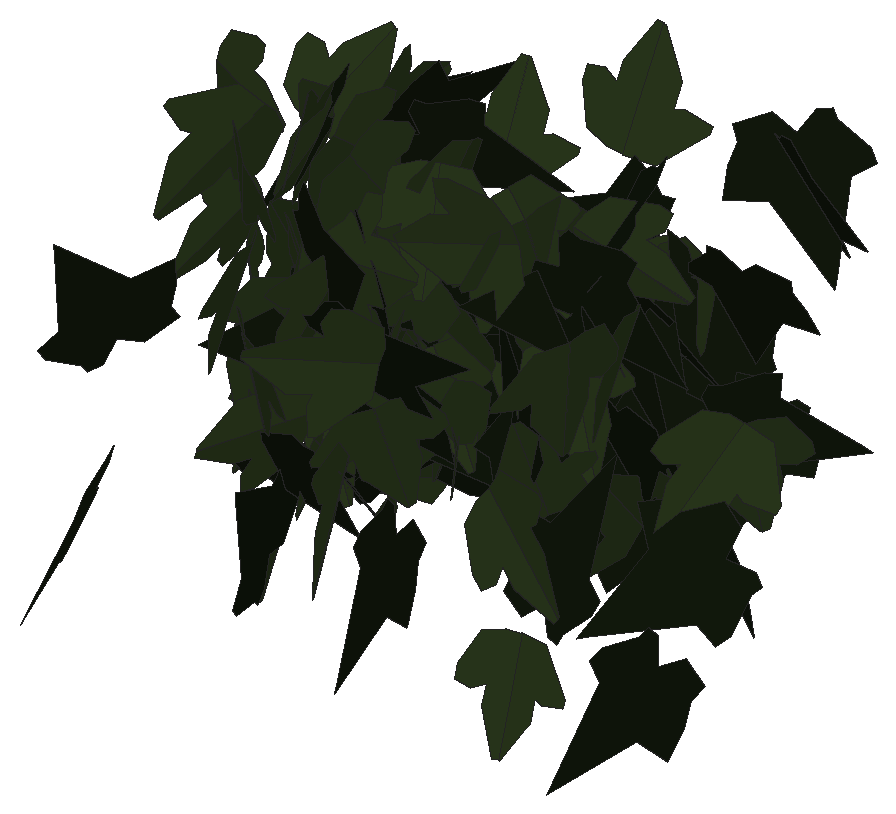
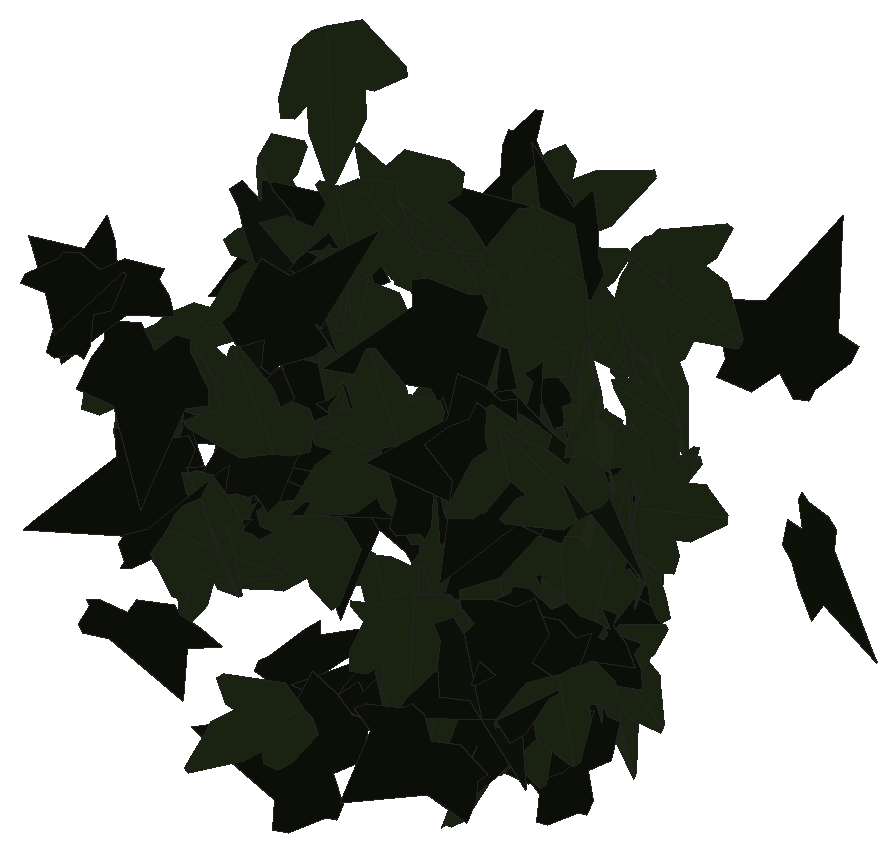
# SketchUp Ruby script. Lengths in inches.
U = 1.inch
M = Sketchup.active_model
def pt(a) = Geom::Point3d.new(a.map { |v| v * U })
def face(e, loops, mat)
  f = e.add_face(loops[0].map { |a| pt(a) })
  loops[1..].each { |l| e.add_face(l.map { |a| pt(a) }).erase! }
  f.material = f.back_material = mat if mat
  f
end
# faces: each face lists its corners as indices into pts; further lists are holes
def faces(e, pts, list, mat = nil) = list.each { |f| face(e, (f[0].is_a?(Array) ? f : [f]).map { |l| l.map { |i| pts[i] } }, mat) }
# xy, xz, yz: faces in a plane at the given z, y or x. An outline is a flat list of corners, or four numbers for a rectangle; further outlines are holes
def ring(l) = l.size == 4 ? [[l[0], l[1]], [l[2], l[1]], [l[2], l[3]], [l[0], l[3]]] : l.each_slice(2).to_a
def flat(e, list, mat, &to3) = list.each { |f| face(e, (f[0].is_a?(Array) ? f : [f]).map { |l| ring(l).map { |u, v| to3.(u, v) } }, mat) }
def xy(e, z, list, mat = nil) = flat(e, list, mat) { |x, y| [x, y, z] }
def xz(e, y, list, mat = nil) = flat(e, list, mat) { |x, z| [x, y, z] }
def yz(e, x, list, mat = nil) = flat(e, list, mat) { |y, z| [x, y, z] }
def lines(e, pts, list) = list.each { |a, b| e.add_line(pt(pts[a]), pt(pts[b])) }
# prism: a flat outline (further loops are holes) pulled along v
def prism(e, loops, v, mat = nil)
  f = face(e, loops, mat); d = Geom::Vector3d.new(v.map { |x| x * U })
  f.pushpull(f.normal.samedirection?(d) ? d.length : -d.length)
end
def box(e, o, s, mat = nil) = prism(e, [[o, [o[0] + s[0], o[1], o[2]], [o[0] + s[0], o[1] + s[1], o[2]], [o[0], o[1] + s[1], o[2]]]], [0, 0, s[2]], mat)
def at(x, y, z, deg = 0) = Geom::Transformation.translation(pt([x, y, z])) * Geom::Transformation.rotation(ORIGIN, Z_AXIS, deg.degrees)
def axes(o, x, y, z) = Geom::Transformation.new([*x, 0, *y, 0, *z, 0, *pt(o).to_a, 1])
def part(name) = M.definitions.add(name)
# library, detail: a bought-in or finely detailed component or shape, given as its bounding box
def library(name, o, s) = part(name).tap { |d| box(d.entities, o, s) }
def detail(e, o, s) = box(e.add_group.entities, o, s)
def put(e, d, t, mat = nil) = e.add_instance(d, t).tap { |i| i.material = mat if mat }
def group(e, t, mat = nil) = e.add_group.tap { |g| g.transformation = t; g.material = mat if mat }.entities
root = M.entities
M.materials.add("efeu1").color = [18, 25, 13]
M.materials.add("efeu2").color = [43, 57, 29]
c1 = part("ivyleaf_10")
p = [[0,0.5,-0.03],[-0.0625,2.02,-0.43],[-0.19,2.01,-0.46],[-0.54,1.05,-0.29],[-0.52,0.625,-0.18],[-0.83,0.76,-0.28],
  [-1.16,0.64,-0.33],[-1.15,0.33,-0.24],[-0.77,-0.39,0.02],[-0.3,-0.51,0.16],[0.04,-0.48,0.23],[-0.02,2.01,-0.4375],
  [-0.06,2.01,-0.43],[0.04,-0.49,0.23],[0.67,-0.49,0.14],[1.38,0.36,-0.2],[1.375,0.51,-0.24],[0.81,0.65,-0.19],
  [0.62,0.59,-0.15],[0.6,1.09,-0.28],[0.5,1.23,-0.31]]
faces(c1.entities,p,[[0,1,2,3,4,5,6,7,8,9,10],[11,12,0,13,14,15,16,17,18,19,20]],"efeu2")
c2 = part("ivyleaf_9")
p = [[1.54,2.16,1.25],[1.36,2.04,1.19],[-0.21,0.99,0.68],[-0.71,1.11,0.82],[-0.85,0.86,0.67],[-0.8,0.17,0.21],
  [-0.9,-0.01,0.1],[-0.67,-0.16,-0.02],[-0.08,-0.08,-0.05],[-0.03,-0.6,-0.4],[0.65,-0.88,-0.66],[0.83,-0.6,-0.49],
  [1.29,-0.42,-0.43],[1.8125,-0.07,-0.26],[1.21,0.44,0.15]]
faces(c2.entities,p,[[0,1,2,3,4,5,6,7,8,9,10,11,12,13,14]],"efeu1")
put(root,c1,axes([532.08,134.94,161.78],[-0.002,-0.30282,0.71041],[0.08269,-0.70641,-0.30089],[0.76782,0.07529,0.03425]))
put(root,c1,axes([531.67,135.35,163.72],[-0.12036,0.03541,-0.73913],[0.60153,-0.43146,-0.11862],[-0.43098,-0.61209,0.04086]))
put(root,c1,axes([532.1875,137.11,159.68],[0.41197,0.62153,-0.13019],[-0.08175,-0.10199,-0.74558],[-0.62974,0.41984,0.01161]))
put(root,c1,axes([532.44,135.95,160.75],[-0.0692,-0.6273,-0.50852],[-0.05873,-0.50512,0.6311],[-0.80539,0.09073,-0.00233]))
put(root,c2,axes([532.82,136.0625,163.02],[-0.57789,0.4659,-0.23379],[0.18175,-0.14706,-0.74231],[-0.48856,-0.6058,0.00039]))
put(root,c1,axes([532.21,136.84,162.81],[0.52698,0.21784,-0.49866],[0.45176,0.21184,0.56996],[0.30336,-0.69389,0.01746]))
put(root,c2,axes([532.9,130.41,159.11],[-0.55637,0.44266,-0.4062],[0.31798,-0.25276,-0.71098],[-0.50974,-0.64082,-0.00016]))
put(root,c1,axes([532.81,135.01,158.96],[0.02058,-0.62016,0.37202],[0.0037,-0.37207,-0.62046],[0.72318,0.01955,-0.00741]))
put(root,c1,axes([532.47,134.8125,161.05],[-0.14719,0.19766,-0.6896],[0.32766,-0.60772,-0.24413],[-0.63816,-0.35762,0.0337]))
put(root,c1,axes([533.27,135.22,160.39],[-0.47943,0.47544,-0.49846],[-0.36513,0.33957,0.67508],[0.58411,0.6025,0.01287]))
put(root,c1,axes([532.75,135.95,162.83],[0.0508,-0.06086,0.8255],[0.40432,-0.71985,-0.07795],[0.72227,0.40725,-0.01442]))
put(root,c1,axes([532.84,135.5,162.92],[0.12973,-0.60881,-0.37491],[0.143,-0.35124,0.61985],[-0.70054,-0.18444,0.0571]))
put(root,c2,axes([533.25,130.55,161.94],[0.37841,0.24051,0.68698],[-0.58544,-0.3595,0.44833],[0.43249,-0.69706,0.00581]))
put(root,c2,axes([532.9,135.89,159.72],[-0.20956,-0.51365,-0.5596],[0.32969,0.46147,-0.54704],[0.68432,-0.37962,0.09218]))
put(root,c2,axes([532.74,137.26,160],[0.68336,0.09355,0.33582],[0.32711,0.08341,-0.68888],[-0.12052,0.75684,0.03441]))
put(root,c1,axes([533.54,133.16,164.47],[-0.21876,-0.59381,0.66253],[-0.17439,-0.64041,-0.63157],[0.87244,-0.27691,0.03988]))
put(root,c1,axes([533.41,136.84,162.85],[0.0594,-0.09073,0.83556],[-0.28118,0.78724,0.10547],[-0.79204,-0.28628,0.02522]))
put(root,c2,axes([533.12,136.14,160.23],[-0.44385,-0.46624,-0.522],[0.35371,0.38395,-0.6437],[0.60395,-0.56751,-0.00664]))
put(root,c2,axes([533.65,137.23,160.01],[-0.29303,0.70506,-0.12806],[0.04388,-0.12045,-0.76351],[-0.71525,-0.29624,0.00563]))
put(root,c2,axes([532.72,135.91,157.64],[0.40534,-0.27587,0.6099],[0.49352,-0.35854,-0.49017],[0.45224,0.63853,-0.01174]))
put(root,c1,axes([532.81,134.05,160.11],[0.10197,-0.05267,0.80903],[0.76764,-0.25606,-0.11342],[0.26083,0.77418,0.01753]))
put(root,c2,axes([533.56,136.77,157.74],[-0.63085,-0.329,0.56453],[0.50052,0.26111,0.71148],[-0.42002,0.80529,-0.00005]))
put(root,c2,axes([533.49,136.75,162.95],[0.26609,0.67068,0.27237],[0.10609,0.25093,-0.72151],[-0.71606,0.2864,-0.00569]))
put(root,c2,axes([533.15,139.05,159.29],[-0.13744,-0.26779,-0.74332],[0.5637,0.49543,-0.28271],[0.55361,-0.57094,0.10332]))
put(root,c1,axes([533.44,136.55,158.5],[-0.58202,-0.00313,-0.44676],[0.44661,0.01584,-0.58193],[0.01213,-0.73355,-0.01066]))
put(root,c1,axes([533.9,133.79,157.9],[0.28195,-0.793,0.06815],[0.02985,-0.06171,-0.8416],[0.79537,0.28342,0.00743]))
put(root,c1,axes([534.27,132.43,164.17],[-0.55254,0.30245,0.48443],[-0.43196,0.2196,-0.62979],[-0.37358,-0.70125,0.01171]))
put(root,c1,axes([534.02,137.2,157.17],[-0.28529,0.625,0.35081],[0.12301,-0.32929,0.68667],[0.70609,0.30989,0.02212]))
put(root,c2,axes([533.8,136.75,162.89],[0.23318,0.16249,0.71968],[0.48675,0.53333,-0.27812],[-0.55445,0.53654,0.05851]))
put(root,c1,axes([534.16,133.71,161.51],[-0.73139,-0.49272,-0.07491],[0.0621,0.04189,-0.88188],[0.4945,-0.73402,-0.00005]))
put(root,c1,axes([534.15,132.37,162.6],[0.29935,-0.80877,0.14102],[0.04631,-0.13323,-0.86239],[0.81967,0.30289,-0.00277]))
put(root,c2,axes([534.48,134.29,160.63],[-0.27299,-0.1747,0.71214],[-0.56109,-0.43945,-0.32289],[0.47207,-0.62334,0.02804]))
put(root,c1,axes([534.28,138.01,160.44],[-0.52586,-0.67296,-0.06046],[0.03666,0.04808,-0.85405],[0.67468,-0.52714,-0.00071]))
put(root,c1,axes([534.46,133.21,161.04],[0.67826,-0.42746,0.19087],[-0.15729,0.10839,0.80169],[-0.44093,-0.69621,0.00762]))
put(root,c1,axes([534.66,135.55,160.18],[-0.18858,-0.72656,0.27632],[-0.06399,-0.26886,-0.75062],[0.77469,-0.19907,0.00526]))
put(root,c1,axes([534.29,135.91,159.06],[0.28461,-0.31504,0.64025],[0.41826,-0.48482,-0.42448],[0.57813,0.50585,-0.00809]))
put(root,c2,axes([534.62,135.95,160.73],[0.01381,-0.26501,-0.72541],[0.26048,-0.68142,0.2539],[-0.72705,-0.24917,0.07719]))
put(root,c1,axes([534.6,132.89,159.93],[-0.00528,0.14021,0.91001],[0.10978,-0.90344,0.13984],[0.91418,0.1093,-0.01154]))
put(root,c1,axes([534.43,134.36,159.39],[0.2255,-0.51053,0.64216],[0.29224,-0.57229,-0.55762],[0.76655,0.36837,0.02368]))
put(root,c2,axes([534.48,132.65,157.76],[0.08676,0.29022,0.86965],[-0.24158,-0.83543,0.3029],[0.8844,-0.25667,-0.00257]))
put(root,c1,axes([534.77,134.11,164.23],[-0.18751,-0.53461,-0.62944],[0.19083,0.59995,-0.56641],[0.80349,-0.26725,-0.01237]))
put(root,c2,axes([534.58,132.51,159.57],[0.75705,0.24599,-0.0584],[-0.05548,-0.01826,-0.79601],[-0.24666,0.75908,-0.00022]))
put(root,c1,axes([534.4,133.84,159.85],[0.69949,0.06896,0.43914],[0.43568,0.05614,-0.70279],[-0.08822,0.824,0.01113]))
put(root,c1,axes([534.83,135.05,162.02],[-0.90639,-0.03716,-0.14843],[0.14883,-0.00695,-0.90706],[0.03555,-0.91843,0.01287]))
put(root,c1,axes([535.03,136.6,158.17],[-0.30064,-0.78217,-0.38143],[-0.12741,-0.35964,0.83791],[-0.86084,0.32639,0.0092]))
put(root,c1,axes([535.2,131.37,161.96],[-0.66871,0.45432,0.25237],[-0.21768,0.12859,-0.80829],[-0.47192,-0.70308,0.01524]))
put(root,c2,axes([534.84,133.91,160.64],[-0.48126,0.14357,0.66024],[0.59014,-0.30542,0.49658],[0.32903,0.75779,0.07505]))
put(root,c1,axes([535.03,135.79,160.85],[-0.32543,-0.51482,-0.62688],[0.3058,0.54776,-0.60859],[0.75134,-0.44592,-0.02383]))
put(root,c1,axes([535.24,136.73,159.22],[0.77108,0.08981,0.09917],[-0.09865,-0.01018,0.77629],[0.09037,-0.77736,0.00129]))
put(root,c1,axes([535.33,136.27,159.28],[0.17943,-0.67412,0.26593],[0.08093,-0.25361,-0.69749],[0.72015,0.19647,0.01212]))
put(root,c2,axes([535.11,135.25,159.74],[0.044,-0.41459,-0.74425],[-0.04672,0.74295,-0.41662],[0.85065,0.06224,0.01562]))
put(root,c2,axes([534.84,136.9,162.02],[0.22896,-0.27836,0.6869],[0.40157,-0.55767,-0.35984],[0.62295,0.4618,-0.0205]))
put(root,c2,axes([535.44,134.11,158.94],[0.30782,0.53031,0.49446],[0.23056,0.4377,-0.61297],[-0.68743,0.38426,0.01583]))
put(root,c1,axes([536.16,135.28,160.5],[-0.39536,0.1074,-0.69101],[-0.67271,0.15841,0.40952],[0.19101,0.7802,0.01197]))
put(root,c1,axes([535.45,137,162.9375],[0.66068,0.34913,-0.17887],[0.15399,0.09142,0.74721],[0.3608,-0.67834,0.00864]))
put(root,c2,axes([534.99,136.09,158.18],[0.48199,0.06136,0.68216],[0.67861,0.07009,-0.48579],[-0.09268,0.83231,-0.00938]))
put(root,c2,axes([535.35,137,159.43],[0.17233,-0.76287,-0.0972],[-0.01989,0.09515,-0.78209],[0.76878,0.17347,0.00155]))
put(root,c2,axes([535.99,133.1,163.11],[0.277,0.05335,-0.76462],[-0.7643,0.08051,-0.27127],[0.05778,0.80925,0.0774]))
put(root,c1,axes([535.25,139.96,159.38],[0.23488,0.3399,0.67518],[0.40679,0.53909,-0.4129],[-0.63713,0.4695,-0.01471]))
put(root,c1,axes([535.79,134.02,160.51],[-0.29563,-0.72009,-0.13796],[0.05596,0.12615,-0.7784],[0.73105,-0.30085,0.00379]))
put(root,c1,axes([535.67,133.33,164.43],[-0.19077,-0.67734,-0.5132],[0.24073,0.46136,-0.6984],[0.815,-0.29482,0.08616]))
put(root,c2,axes([535.25,135.42,163.85],[0.12935,0.15181,-0.77032],[0.41543,0.64923,0.1977],[0.66623,-0.4343,0.02628]))
put(root,c1,axes([535.92,132.26,162.98],[-0.01678,-0.71517,0.4305],[-0.01843,-0.43017,-0.71533],[0.83454,-0.02388,-0.00714]))
put(root,c1,axes([535.78,133.65,160.64],[0.4631,-0.67856,0.1728],[-0.05838,0.16904,0.82023],[-0.69778,-0.46449,0.04606]))
put(root,c1,axes([536.38,133.94,162.32],[-0.37144,-0.14663,0.6472],[-0.56878,-0.31172,-0.39705],[0.34184,-0.67799,0.04258]))
put(root,c2,axes([535.37,138.67,157.875],[0.44281,-0.17669,0.66191],[0.62981,-0.20514,-0.4761],[0.26958,0.76949,0.02506]))
put(root,c2,axes([535.75,135.31,161.56],[0.1156,0.14244,-0.8342],[0.2386,0.8023,0.17006],[0.81194,-0.25605,0.06879]))
put(root,c1,axes([536.26,134.9,164.02],[0.0995,-0.7101,0.29811],[0.02913,-0.2969,-0.71694],[0.76958,0.10304,-0.01141]))
put(root,c1,axes([535.55,133.15,162.91],[0.13255,-0.19964,-0.90011],[0.78454,-0.45326,0.21606],[-0.48431,-0.78888,0.10365]))
put(root,c2,axes([535.77,136.06,160.78],[-0.10007,0.15743,0.80572],[0.51659,-0.61876,0.18506],[0.63804,0.52568,-0.02346]))
put(root,c2,axes([535.84,132.21,163.17],[0.01991,-0.07783,0.86073],[0.39433,-0.7653,-0.07832],[0.76904,0.39442,0.01787]))
put(root,c2,axes([536.69,132.64,161.38],[0.47463,0.30534,-0.65791],[-0.57799,-0.31578,-0.56353],[-0.43819,0.74726,0.03069]))
put(root,c1,axes([536.43,134.12,163.91],[0.77574,0.29292,-0.00672],[-0.00626,-0.00244,-0.8292],[-0.29293,0.77577,-0.00007]))
put(root,c1,axes([536.375,136.15,161.85],[-0.54697,-0.18962,-0.59795],[0.5688,0.18461,-0.57885],[0.26452,-0.78908,0.00826]))
put(root,c1,axes([536.6,138.61,163.12],[0.76257,0.24788,-0.21122],[0.20122,0.06424,0.80184],[0.25606,-0.78867,-0.00107]))
put(root,c2,axes([536.68,132.14,159.63],[0.64329,-0.43889,-0.06623],[0.06083,-0.02835,0.77867],[-0.43967,-0.64607,0.01082]))
put(root,c1,axes([536.67,132.67,158.81],[0.30413,-0.34575,0.73459],[0.48369,-0.55287,-0.46047],[0.65207,0.57136,-0.00105]))
put(root,c1,axes([537.34,133.17,161.13],[-0.44568,-0.63806,0.41851],[-0.20978,-0.36353,-0.77765],[0.73366,-0.49155,0.03187]))
put(root,c1,axes([536.65,133.96,160.99],[0.61334,0.0572,0.44802],[0.44678,0.03384,-0.61597],[-0.06616,0.75879,-0.0063]))
put(root,c1,axes([536.77,134.21,159.84],[-0.21521,0.17067,0.69672],[0.5486,-0.42948,0.27466],[0.46214,0.5893,-0.0016]))
put(root,c1,axes([537.26,131.83,161.24],[-0.53005,-0.61644,-0.22224],[0.15053,0.16365,-0.81296],[0.63775,-0.55097,0.00718]))
put(root,c1,axes([537.67,130.66,162.93],[-0.12192,-0.13674,-0.84716],[-0.613,-0.5849,0.18263],[-0.6005,0.62484,-0.01444]))
put(root,c1,axes([537.3125,130.71,160.75],[0.25101,-0.50253,0.66321],[0.42763,-0.51635,-0.55309],[0.71381,0.48605,0.09813]))
put(root,c2,axes([537.75,137.03,157.91],[0.08059,-0.52699,-0.60206],[0.07232,-0.59783,0.53297],[-0.79684,-0.10755,-0.01252]))
put(root,c2,axes([536.87,131.51,162.54],[0.68304,0.23669,-0.56849],[0.53466,0.19327,0.72287],[0.30552,-0.86739,0.00594]))
put(root,c1,axes([538.3,133.11,164.1],[0.3403,-0.06903,-0.8921],[-0.85331,0.2621,-0.34578],[0.26918,0.91812,0.03164]))
put(root,c1,axes([537.43,136.28,160.09],[-0.32249,-0.23513,-0.68343],[0.58973,0.34705,-0.39768],[0.41784,-0.6713,0.03379]))
put(root,c2,axes([537.96,135.01,160.67],[0.27239,0.73506,-0.23254],[-0.09045,-0.21445,-0.78384],[-0.76564,0.28685,0.00987]))
put(root,c1,axes([538.28,138.28,160.67],[0.29324,0.25277,-0.66649],[-0.5712,-0.34779,-0.38322],[-0.42641,0.63972,0.055]))
put(root,c1,axes([538.21,138.07,161.29],[0.58114,-0.3353,-0.37151],[-0.30331,0.21687,-0.67018],[0.39806,0.65476,0.03173]))
put(root,c1,axes([538.33,134.24,162.71],[-0.84906,-0.21455,-0.05141],[0.05141,0.00638,-0.87573],[0.21455,-0.85059,0.0064]))
put(root,c2,axes([538.7,133.43,160.46],[0.04873,-0.06134,0.83268],[-0.27621,0.78595,0.07406],[-0.78793,-0.27931,0.02553]))
put(root,c2,axes([538.62,136,162.97],[0.02562,0.00766,0.76909],[-0.60333,-0.47707,0.02485],[0.47703,-0.60379,-0.00988]))
put(root,c2,axes([537.99,136.6,161.8],[0.78639,-0.14682,0.00051],[0.00114,0.00332,-0.79997],[0.14682,0.78638,0.00347]))
put(root,c1,axes([538.56,133.72,164.09],[-0.34013,-0.76932,-0.27925],[0.13426,0.24586,-0.84086],[0.80735,-0.365,0.02219]))
put(root,c1,axes([538.06,134.09,164.1],[0.59498,0.15305,0.53597],[0.5235,0.1158,-0.61419],[-0.19143,0.79237,-0.01377]))
put(root,c2,axes([538.35,134.3125,160.67],[-0.00531,-0.24572,-0.8413],[0.03549,0.84057,-0.24573],[0.87573,-0.03555,0.00485]))
put(root,c2,axes([538.95,138.07,160.09],[-0.47588,-0.57984,0.17724],[0.11312,0.13644,0.75012],[-0.59568,0.48914,0.00086]))
put(root,c2,axes([538.53,134.55,161.0625],[-0.04016,0.37404,-0.69863],[-0.16862,0.67948,0.37347],[0.77431,0.16737,0.04509]))
put(root,c2,axes([539.17,134.66,162.63],[-0.25289,-0.14558,0.80927],[-0.57926,-0.56937,-0.28344],[0.58358,-0.62824,0.06935]))
put(root,c2,axes([538.92,135.79,160.04],[-0.65653,0.00947,0.4012],[0.40127,0.00463,0.65654],[0.00567,0.7694,-0.00889]))
put(root,c1,axes([539.09,133.43,159.92],[-0.44524,-0.63436,-0.32306],[-0.18102,-0.26763,0.775],[-0.68849,0.4806,0.00515]))
put(root,c1,axes([538.98,132.83,157.42],[0.77796,0.01551,0.01079],[0.01074,0.00255,-0.77811],[-0.01555,0.77803,0.00233]))
put(root,c2,axes([539.17,138.57,159.13],[-0.62363,-0.41385,-0.21587],[0.1793,0.12022,-0.74846],[0.43096,-0.64889,-0.00098]))
put(root,c2,axes([539.61,134.86,164.26],[-0.5425,0.62115,-0.0616],[0.04001,-0.04685,-0.82471],[-0.62292,-0.54398,0.00068]))
put(root,c1,axes([538.95,134.87,163.67],[-0.48694,-0.30004,-0.64164],[0.58338,0.27173,-0.56979],[0.40174,-0.75827,0.0497]))
put(root,c1,axes([539.34,135.35,158.84],[-0.17202,-0.60054,-0.57502],[-0.09219,-0.5698,0.62267],[-0.82632,0.18859,0.05024]))
put(root,c1,axes([538.98,134.12,161.85],[0.78758,0.11324,0.37942],[0.37652,0.04721,-0.79566],[-0.12254,0.87293,-0.00619]))
put(root,c2,axes([539.08,133.92,163.56],[-0.06431,-0.04493,-0.85682],[0.61524,0.59647,-0.07746],[0.59803,-0.61846,-0.01246]))
put(root,c2,axes([539.18,134.91,162.53],[0.45698,-0.68723,0.10637],[0.05611,-0.09042,-0.82529],[0.69315,0.4604,-0.00332]))
put(root,c1,axes([539.77,136,159.14],[-0.00311,-0.52012,-0.61428],[-0.0287,0.61397,-0.51971],[0.80439,0.0199,-0.02092]))
put(root,c2,axes([539.75,134.4,161.14],[0.62329,0.16239,-0.47769],[-0.46739,-0.10012,-0.64388],[-0.19003,0.77888,0.01683]))
put(root,c2,axes([540.05,136.95,162.51],[0.55494,0.30479,-0.44667],[-0.39709,-0.20476,-0.63306],[-0.36706,0.68231,0.00955]))
put(root,c2,axes([539.98,136.46,160.21],[0.13291,0.17433,-0.78554],[0.20034,0.76394,0.20343],[0.77931,-0.22612,0.08167]))
put(root,c2,axes([540.21,128.45,161.76],[-0.05409,0.05349,-0.87386],[0.62484,-0.6109,-0.07607],[-0.61324,-0.62718,-0.00043]))
put(root,c2,axes([540.18,138.08,164.375],[-0.27749,-0.53271,-0.5056],[0.26273,0.43271,-0.60011],[0.68584,-0.3813,0.02533]))
put(root,c1,axes([540.9,133.07,163.51],[0.32133,-0.73321,0.24571],[0.0983,-0.22519,-0.80053],[0.76701,0.33603,-0.00034]))
put(root,c2,axes([540.38,138.03,163.65],[0.24987,-0.3492,0.65781],[0.39839,-0.52355,-0.42926],[0.62924,0.47015,0.01057]))
put(root,c2,axes([541.375,134.75,159.47],[0.40733,0.01432,-0.74102],[-0.74114,0.00184,-0.40736],[-0.00529,0.84559,0.01343]))
put(root,c1,axes([540.8125,130.17,161.65],[0.49696,-0.03874,0.73645],[0.7372,0.00195,-0.49736],[0.02005,0.88844,0.0332]))
put(root,c1,axes([541.5,135.16,160.96],[-0.61754,-0.59334,-0.12628],[0.09105,0.0875,-0.85639],[0.59976,-0.62421,-0.00002]))
put(root,c1,axes([541.65,134.55,161.2],[0.56121,0.4258,-0.46867],[-0.37543,-0.28056,-0.70446],[-0.50991,0.67521,0.00284]))
put(root,c1,axes([541.62,130.78,164.3125],[-0.25228,-0.88779,-0.08894],[0.02818,0.08445,-0.92293],[0.89179,-0.25382,0.00401]))
put(root,c2,axes([541.96,133.99,159.63],[-0.67514,-0.29658,0.36083],[-0.33267,-0.13984,-0.7374],[0.32785,-0.75264,-0.00518]))
put(root,c2,axes([541.38,130.62,160.28],[-0.50663,0.52755,0.4739],[0.31622,-0.35324,0.73129],[0.63474,0.59705,0.01393]))
put(root,c2,axes([541.6,132.89,158.09],[-0.0192,0.00933,-0.83943],[0.28832,-0.7885,-0.01536],[-0.78842,-0.28858,0.01482]))
